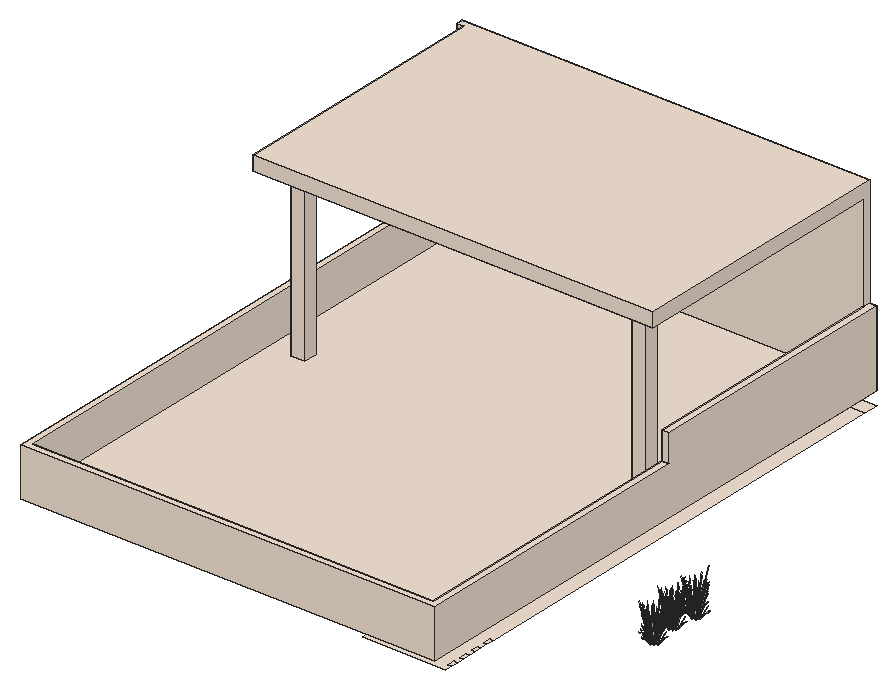
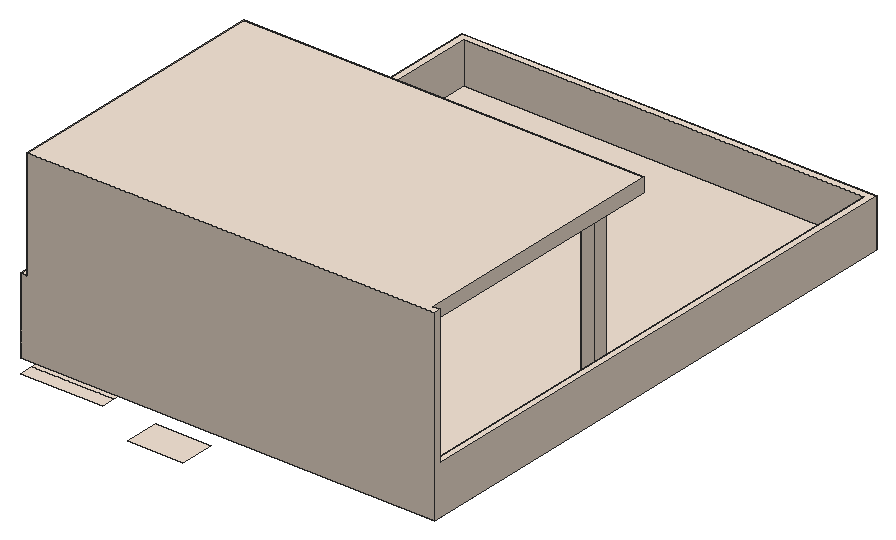
# SketchUp Ruby script. Lengths in inches.
U = 1.inch
M = Sketchup.active_model
def pt(a) = Geom::Point3d.new(a.map { |v| v * U })
def face(e, loops, mat)
  f = e.add_face(loops[0].map { |a| pt(a) })
  loops[1..].each { |l| e.add_face(l.map { |a| pt(a) }).erase! }
  f.material = f.back_material = mat if mat
  f
end
# faces: each face lists its corners as indices into pts; further lists are holes
def faces(e, pts, list, mat = nil) = list.each { |f| face(e, (f[0].is_a?(Array) ? f : [f]).map { |l| l.map { |i| pts[i] } }, mat) }
# xy, xz, yz: faces in a plane at the given z, y or x. An outline is a flat list of corners, or four numbers for a rectangle; further outlines are holes
def ring(l) = l.size == 4 ? [[l[0], l[1]], [l[2], l[1]], [l[2], l[3]], [l[0], l[3]]] : l.each_slice(2).to_a
def flat(e, list, mat, &to3) = list.each { |f| face(e, (f[0].is_a?(Array) ? f : [f]).map { |l| ring(l).map { |u, v| to3.(u, v) } }, mat) }
def xy(e, z, list, mat = nil) = flat(e, list, mat) { |x, y| [x, y, z] }
def xz(e, y, list, mat = nil) = flat(e, list, mat) { |x, z| [x, y, z] }
def yz(e, x, list, mat = nil) = flat(e, list, mat) { |y, z| [x, y, z] }
def lines(e, pts, list) = list.each { |a, b| e.add_line(pt(pts[a]), pt(pts[b])) }
# prism: a flat outline (further loops are holes) pulled along v
def prism(e, loops, v, mat = nil)
  f = face(e, loops, mat); d = Geom::Vector3d.new(v.map { |x| x * U })
  f.pushpull(f.normal.samedirection?(d) ? d.length : -d.length)
end
def box(e, o, s, mat = nil) = prism(e, [[o, [o[0] + s[0], o[1], o[2]], [o[0] + s[0], o[1] + s[1], o[2]], [o[0], o[1] + s[1], o[2]]]], [0, 0, s[2]], mat)
def at(x, y, z, deg = 0) = Geom::Transformation.translation(pt([x, y, z])) * Geom::Transformation.rotation(ORIGIN, Z_AXIS, deg.degrees)
def axes(o, x, y, z) = Geom::Transformation.new([*x, 0, *y, 0, *z, 0, *pt(o).to_a, 1])
def part(name) = M.definitions.add(name)
# library, detail: a bought-in or finely detailed component or shape, given as its bounding box
def library(name, o, s) = part(name).tap { |d| box(d.entities, o, s) }
def detail(e, o, s) = box(e.add_group.entities, o, s)
def put(e, d, t, mat = nil) = e.add_instance(d, t).tap { |i| i.material = mat if mat }
def group(e, t, mat = nil) = e.add_group.tap { |g| g.transformation = t; g.material = mat if mat }.entities
root = M.entities
M.materials.add("C01_Vanilla_Cream").color = [244, 228, 212]
M.materials.add("LightPink_Translucent").color = [144, 107, 117]
M.materials["LightPink_Translucent"].alpha = 0.75
c1 = part("blade")
p = [[2.15,0.21,22],[0,0.17,0],[0.09,0.45,0],[2.18,0.31,22],[2.29,0.31,22],[0.38,0.45,0],
  [2.48,0.24,33],[2.49,0.24,33],[2.48,0.22,33]]
faces(c1.entities,p,[[0,1,2,3],[4,5,2,3],[6,3,4,7],[8,0,3,6]])
c2 = part("seeds")
p = [[0.3,-0.1,1.38],[-0.01,-0.03,1.59],[-0.01,-0.03,0.03],[0.14,-0.07,-0.07],[0.29,-0.03,3],[0.15,0.01,3.11]]
faces(c2.entities,p,[[0,1,2,3],[1,0,4,5]],"LightPink_Translucent")
c3 = part("blade with seeds")
put(c3.entities,c1,at(0,0,0))
put(c3.entities,c2,axes([2.4,0.25,30.99],[1.5799,-0.05474,1.17369],[-0.12525,1.92788,0.29478],[-0.07173,-0.02425,1.56792]))
xy(root,543,[[226.53,171,288,201],[240,327,290,358.5],[240,361.5,290,393],[240,423,288,453]],"C01_Vanilla_Cream")
xy(root,546,[[288,324,290,396]],"C01_Vanilla_Cream")
xy(root,582,[[288,12,288,216,326.85,216,326.85,314.71,288,314.71,288,468,360,468,360,63.65,357,63.65,357,57.2,360,57.2,360,50.74,357,50.74,357,44.28,360,44.28,360,37.83,357,37.83,357,31.37,360,31.37,360,24.91,357,24.91,357,18.46,360,18.46,360,12],[357,18.46,360,24.91],[357,31.37,360,37.83],[357,44.28,360,50.74],[357,57.2,360,63.65],
  [288,468,360,480]],"C01_Vanilla_Cream")
xy(root,594,[[[0,0,360,480],[9,9,351,471]]],"C01_Vanilla_Cream")
p = [[360,254.66,636],[354,254.66,636]]
lines(root,p,[[0,1]])
put(root,c3,axes([356.1,285.38,501.78],[-0.02981,0.50103,-0.0912],[-0.56442,-0.01369,-0.50621],[-0.21738,-0.0348,0.76918]))
put(root,c3,axes([358.58,288.78,501.78],[0.33176,-0.4217,-0.0912],[0.48044,0.24295,-0.50621],[0.16701,0.11914,0.76918]))
put(root,c3,axes([355.49,287.37,501.78],[0.515,0.27165,-0.0912],[-0.2967,0.3934,-0.50621],[-0.1455,0.13675,0.76918]))
put(root,c3,axes([358.5,284.82,501.78],[-0.54481,0.22937,-0.0912],[-0.26773,-0.4071,-0.50621],[-0.07188,-0.17155,0.76918]))
put(root,c3,axes([360.3,286.25,501.78],[-0.515,-0.27165,-0.0912],[0.2967,-0.3934,-0.50621],[0.1455,-0.13675,0.76918]))
put(root,c3,axes([358.96,240.81,501.36],[-0.48108,-0.25598,1.03712],[0.50798,-0.39855,0.44749],[0.15521,0.24018,1.00248]))
put(root,c3,axes([355.92,264.77,501.36],[-0.48108,-0.25598,1.03712],[0.50798,-0.39855,0.44749],[0.15521,0.24018,1.00248]))
put(root,c3,axes([358.96,286.29,501.36],[-0.48108,-0.25598,1.03712],[0.50798,-0.39855,0.44749],[0.15521,0.24018,1.00248]))
put(root,c3,axes([354.88,241.27,501.54],[-0.09091,0.06396,1.31208],[0.00773,0.46734,-0.2075],[-0.20839,0.06078,0.10523]))
put(root,c3,axes([361.84,241.125,501.54],[0.07726,-0.07504,1.31208],[-0.09888,-0.46032,-0.2075],[0.19384,-0.08728,0.10523]))
put(root,c3,axes([360.18,242.45,501.54],[0.11943,-0.00833,1.31208],[0.32759,-0.38275,-0.2075],[0.21244,0.05052,0.10523]))
put(root,c3,axes([360.19,239.12,501.54],[-0.00537,-0.09805,1.31208],[-0.45391,-0.28338,-0.2075],[0.07018,-0.17178,0.10523]))
put(root,c3,axes([354.9,243.02,501.54],[-0.01384,0.09749,1.31208],[0.39274,0.33916,-0.2075],[-0.10282,0.16039,0.10523]))
put(root,c3,axes([357.16,244.22,501.54],[0.07057,0.07933,1.31208],[0.56952,0.03117,-0.2075],[0.05727,0.17496,0.10523]))
put(root,c3,axes([357.64,238.27,501.54],[-0.08515,-0.06907,1.31208],[-0.56828,0.04379,-0.2075],[-0.0907,-0.16522,0.10523]))
put(root,c3,axes([355.77,239.03,501.54],[-0.11979,-0.00348,1.31208],[-0.38137,0.34775,-0.2075],[-0.20349,-0.07106,0.10523]))
put(root,c3,axes([351.85,265.24,501.54],[-0.09091,0.06396,1.31208],[0.00773,0.46734,-0.2075],[-0.20839,0.06078,0.10523]))
put(root,c3,axes([358.8,265.09,501.54],[0.07726,-0.07504,1.31208],[-0.09888,-0.46032,-0.2075],[0.19384,-0.08728,0.10523]))
put(root,c3,axes([357.14,266.42,501.54],[0.11943,-0.00833,1.31208],[0.32759,-0.38275,-0.2075],[0.21244,0.05052,0.10523]))
put(root,c3,axes([357.15,263.08,501.54],[-0.00537,-0.09805,1.31208],[-0.45391,-0.28338,-0.2075],[0.07018,-0.17178,0.10523]))
put(root,c3,axes([351.86,266.98,501.54],[-0.01384,0.09749,1.31208],[0.39274,0.33916,-0.2075],[-0.10282,0.16039,0.10523]))
put(root,c3,axes([354.12,268.1875,501.54],[0.07057,0.07933,1.31208],[0.56952,0.03117,-0.2075],[0.05727,0.17496,0.10523]))
put(root,c3,axes([354.6,262.24,501.54],[-0.08515,-0.06907,1.31208],[-0.56828,0.04379,-0.2075],[-0.0907,-0.16522,0.10523]))
put(root,c3,axes([352.74,263,501.54],[-0.11979,-0.00348,1.31208],[-0.38137,0.34775,-0.2075],[-0.20349,-0.07106,0.10523]))
put(root,c3,axes([354.88,286.76,501.54],[-0.09091,0.06396,1.31208],[0.00773,0.46734,-0.2075],[-0.20839,0.06078,0.10523]))
put(root,c3,axes([361.84,286.61,501.54],[0.07726,-0.07504,1.31208],[-0.09888,-0.46032,-0.2075],[0.19384,-0.08728,0.10523]))
put(root,c3,axes([360.18,287.93,501.54],[0.11943,-0.00833,1.31208],[0.32759,-0.38275,-0.2075],[0.21244,0.05052,0.10523]))
put(root,c3,axes([360.19,284.6,501.54],[-0.00537,-0.09805,1.31208],[-0.45391,-0.28338,-0.2075],[0.07018,-0.17178,0.10523]))
put(root,c3,axes([354.9,288.5,501.54],[-0.01384,0.09749,1.31208],[0.39274,0.33916,-0.2075],[-0.10282,0.16039,0.10523]))
put(root,c3,axes([357.16,289.71,501.54],[0.07057,0.07933,1.31208],[0.56952,0.03117,-0.2075],[0.05727,0.17496,0.10523]))
put(root,c3,axes([357.64,283.76,501.54],[-0.08515,-0.06907,1.31208],[-0.56828,0.04379,-0.2075],[-0.0907,-0.16522,0.10523]))
put(root,c3,axes([355.77,284.52,501.54],[-0.11979,-0.00348,1.31208],[-0.38137,0.34775,-0.2075],[-0.20349,-0.07106,0.10523]))
put(root,c3,axes([355.3125,239.33,501.53],[0.04127,0.04917,1.33037],[-0.19898,0.44196,-0.12571],[-0.20151,0.0032,0.23543]))
put(root,c3,axes([357.05,238.05,501.53],[-0.01039,0.05905,1.33037],[-0.51226,0.21431,-0.12571],[-0.15074,-0.10955,0.23543]))
put(root,c3,axes([358.15,243.64,501.53],[0.00165,-0.05965,1.33037],[0.47711,-0.26315,-0.12571],[0.16572,0.09393,0.23543]))
put(root,c3,axes([353.87,241.74,501.53],[0.07105,0.01321,1.33037],[0.2198,0.43529,-0.12571],[-0.14545,0.11425,0.23543]))
put(root,c3,axes([361.57,240.64,501.53],[-0.07272,-0.00374,1.33037],[-0.30197,-0.40092,-0.12571],[0.12127,-0.13182,0.23543]))
put(root,c3,axes([361.44,243.15,501.53],[-0.05034,-0.04313,1.33037],[0.11012,-0.46232,-0.12571],[0.1983,-0.02954,0.23543]))
put(root,c3,axes([354.85,244.02,501.53],[0.06316,-0.02974,1.33037],[0.52204,0.19785,-0.12571],[-0.01227,0.16473,0.23543]))
put(root,c3,axes([360.07,238.77,501.53],[-0.05654,0.03763,1.33037],[-0.55396,-0.12696,-0.12571],[-0.02005,-0.16422,0.23543]))
put(root,c3,axes([352.28,263.29,501.53],[0.04127,0.04917,1.33037],[-0.19898,0.44196,-0.12571],[-0.20151,0.0032,0.23543]))
put(root,c3,axes([354.02,262.01,501.53],[-0.01039,0.05905,1.33037],[-0.51226,0.21431,-0.12571],[-0.15074,-0.10955,0.23543]))
put(root,c3,axes([355.11,267.61,501.53],[0.00165,-0.05965,1.33037],[0.47711,-0.26315,-0.12571],[0.16572,0.09393,0.23543]))
put(root,c3,axes([350.84,265.71,501.53],[0.07105,0.01321,1.33037],[0.2198,0.43529,-0.12571],[-0.14545,0.11425,0.23543]))
put(root,c3,axes([358.53,264.61,501.53],[-0.07272,-0.00374,1.33037],[-0.30197,-0.40092,-0.12571],[0.12127,-0.13182,0.23543]))
put(root,c3,axes([358.4,267.11,501.53],[-0.05034,-0.04313,1.33037],[0.11012,-0.46232,-0.12571],[0.1983,-0.02954,0.23543]))
put(root,c3,axes([351.82,267.98,501.53],[0.06316,-0.02974,1.33037],[0.52204,0.19785,-0.12571],[-0.01227,0.16473,0.23543]))
put(root,c3,axes([357.03,262.73,501.53],[-0.05654,0.03763,1.33037],[-0.55396,-0.12696,-0.12571],[-0.02005,-0.16422,0.23543]))
put(root,c3,axes([355.3125,284.8125,501.53],[0.04127,0.04917,1.33037],[-0.19898,0.44196,-0.12571],[-0.20151,0.0032,0.23543]))
put(root,c3,axes([357.05,283.53,501.53],[-0.01039,0.05905,1.33037],[-0.51226,0.21431,-0.12571],[-0.15074,-0.10955,0.23543]))
put(root,c3,axes([358.15,289.13,501.53],[0.00165,-0.05965,1.33037],[0.47711,-0.26315,-0.12571],[0.16572,0.09393,0.23543]))
put(root,c3,axes([353.87,287.23,501.53],[0.07105,0.01321,1.33037],[0.2198,0.43529,-0.12571],[-0.14545,0.11425,0.23543]))
put(root,c3,axes([361.57,286.13,501.53],[-0.07272,-0.00374,1.33037],[-0.30197,-0.40092,-0.12571],[0.12127,-0.13182,0.23543]))
put(root,c3,axes([361.44,288.63,501.53],[-0.05034,-0.04313,1.33037],[0.11012,-0.46232,-0.12571],[0.1983,-0.02954,0.23543]))
put(root,c3,axes([354.85,289.5,501.53],[0.06316,-0.02974,1.33037],[0.52204,0.19785,-0.12571],[-0.01227,0.16473,0.23543]))
put(root,c3,axes([360.07,284.25,501.53],[-0.05654,0.03763,1.33037],[-0.55396,-0.12696,-0.12571],[-0.02005,-0.16422,0.23543]))
put(root,c3,axes([356.15,242.8,502.05],[0.61188,0.02441,-0.10123],[-0.01672,0.46217,-0.56189],[-0.0425,0.178,0.85379]))
put(root,c3,axes([353.12,266.76,502.05],[0.61188,0.02441,-0.10123],[-0.01672,0.46217,-0.56189],[-0.0425,0.178,0.85379]))
put(root,c3,axes([356.15,288.28,502.05],[0.61188,0.02441,-0.10123],[-0.01672,0.46217,-0.56189],[-0.0425,0.178,0.85379]))
put(root,c3,axes([357.2,239.17,502.07],[-0.37157,0.4723,-0.10215],[-0.5381,-0.2721,-0.56695],[-0.18705,-0.13344,0.86148]))
put(root,c3,axes([354.16,263.13,502.07],[-0.37157,0.4723,-0.10215],[-0.5381,-0.2721,-0.56695],[-0.18705,-0.13344,0.86148]))
put(root,c3,axes([357.2,284.65,502.07],[-0.37157,0.4723,-0.10215],[-0.5381,-0.2721,-0.56695],[-0.18705,-0.13344,0.86148]))
put(root,c3,axes([357.08,239.2,501.55],[0.25304,-0.31296,0.04823],[0.36033,0.18221,0.37966],[-0.11649,-0.10034,0.57892]))
put(root,c3,axes([357.3,243.5,501.55],[-0.41024,0.16744,0.04823],[-0.2008,-0.30532,0.37966],[0.03962,0.13459,0.57892]))
put(root,c3,axes([360.49,240.66,501.55],[0.3822,0.20719,0.04823],[-0.22252,0.29505,0.37966],[0.12254,-0.09539,0.57892]))
put(root,c3,axes([360.55,241.8125,501.55],[0.20448,0.33592,0.04823],[-0.37288,0.16442,0.37966],[0.16437,-0.03244,0.57892]))
put(root,c3,axes([355.9,239.82,501.55],[0.02803,-0.37463,0.04823],[0.42332,0.01027,0.37966],[-0.16216,-0.0392,0.57892]))
put(root,c3,axes([359.74,239.6875,501.55],[0.45752,0.02296,0.04823],[-0.01254,0.34663,0.37966],[0.04787,-0.13278,0.57892]))
put(root,c3,axes([359.89,242.83,501.55],[-0.02803,0.37463,0.04823],[-0.42332,-0.01027,0.37966],[0.16216,0.0392,0.57892]))
put(root,c3,axes([355.3,241.99,501.55],[-0.3822,-0.20719,0.04823],[0.22252,-0.29505,0.37966],[-0.12254,0.09539,0.57892]))
put(root,c3,axes([358.49,239.15,501.55],[0.41024,-0.16744,0.04823],[0.2008,0.30532,0.37966],[-0.03962,-0.13459,0.57892]))
put(root,c3,axes([355.24,240.84,501.55],[-0.20448,-0.33592,0.04823],[0.37288,-0.16442,0.37966],[-0.16437,0.03244,0.57892]))
put(root,c3,axes([358.7,243.45,501.55],[-0.25304,0.31296,0.04823],[-0.36033,-0.18221,0.37966],[0.11649,0.10034,0.57892]))
put(root,c3,axes([356.05,242.96,501.55],[-0.45752,-0.02296,0.04823],[0.01254,-0.34663,0.37966],[-0.04787,0.13278,0.57892]))
put(root,c3,axes([354.05,263.17,501.55],[0.25304,-0.31296,0.04823],[0.36033,0.18221,0.37966],[-0.11649,-0.10034,0.57892]))
put(root,c3,axes([354.26,267.46,501.55],[-0.41024,0.16744,0.04823],[-0.2008,-0.30532,0.37966],[0.03962,0.13459,0.57892]))
put(root,c3,axes([357.45,264.63,501.55],[0.3822,0.20719,0.04823],[-0.22252,0.29505,0.37966],[0.12254,-0.09539,0.57892]))
put(root,c3,axes([357.51,265.78,501.55],[0.20448,0.33592,0.04823],[-0.37288,0.16442,0.37966],[0.16437,-0.03244,0.57892]))
put(root,c3,axes([352.86,263.78,501.55],[0.02803,-0.37463,0.04823],[0.42332,0.01027,0.37966],[-0.16216,-0.0392,0.57892]))
put(root,c3,axes([356.7,263.66,501.55],[0.45752,0.02296,0.04823],[-0.01254,0.34663,0.37966],[0.04787,-0.13278,0.57892]))
put(root,c3,axes([356.85,266.8,501.55],[-0.02803,0.37463,0.04823],[-0.42332,-0.01027,0.37966],[0.16216,0.0392,0.57892]))
put(root,c3,axes([352.26,265.95,501.55],[-0.3822,-0.20719,0.04823],[0.22252,-0.29505,0.37966],[-0.12254,0.09539,0.57892]))
put(root,c3,axes([355.45,263.12,501.55],[0.41024,-0.16744,0.04823],[0.2008,0.30532,0.37966],[-0.03962,-0.13459,0.57892]))
put(root,c3,axes([352.21,264.8,501.55],[-0.20448,-0.33592,0.04823],[0.37288,-0.16442,0.37966],[-0.16437,0.03244,0.57892]))
put(root,c3,axes([355.67,267.42,501.55],[-0.25304,0.31296,0.04823],[-0.36033,-0.18221,0.37966],[0.11649,0.10034,0.57892]))
put(root,c3,axes([353.01,266.93,501.55],[-0.45752,-0.02296,0.04823],[0.01254,-0.34663,0.37966],[-0.04787,0.13278,0.57892]))
put(root,c3,axes([357.08,284.69,501.55],[0.25304,-0.31296,0.04823],[0.36033,0.18221,0.37966],[-0.11649,-0.10034,0.57892]))
put(root,c3,axes([357.3,288.98,501.55],[-0.41024,0.16744,0.04823],[-0.2008,-0.30532,0.37966],[0.03962,0.13459,0.57892]))
put(root,c3,axes([360.49,286.15,501.55],[0.3822,0.20719,0.04823],[-0.22252,0.29505,0.37966],[0.12254,-0.09539,0.57892]))
put(root,c3,axes([360.55,287.3,501.55],[0.20448,0.33592,0.04823],[-0.37288,0.16442,0.37966],[0.16437,-0.03244,0.57892]))
put(root,c3,axes([355.9,285.3,501.55],[0.02803,-0.37463,0.04823],[0.42332,0.01027,0.37966],[-0.16216,-0.0392,0.57892]))
put(root,c3,axes([359.74,285.17,501.55],[0.45752,0.02296,0.04823],[-0.01254,0.34663,0.37966],[0.04787,-0.13278,0.57892]))
put(root,c3,axes([359.89,288.32,501.55],[-0.02803,0.37463,0.04823],[-0.42332,-0.01027,0.37966],[0.16216,0.0392,0.57892]))
put(root,c3,axes([355.3,287.47,501.55],[-0.3822,-0.20719,0.04823],[0.22252,-0.29505,0.37966],[-0.12254,0.09539,0.57892]))
put(root,c3,axes([358.49,284.64,501.55],[0.41024,-0.16744,0.04823],[0.2008,0.30532,0.37966],[-0.03962,-0.13459,0.57892]))
put(root,c3,axes([355.24,286.32,501.55],[-0.20448,-0.33592,0.04823],[0.37288,-0.16442,0.37966],[-0.16437,0.03244,0.57892]))
put(root,c3,axes([358.7,288.93,501.55],[-0.25304,0.31296,0.04823],[-0.36033,-0.18221,0.37966],[0.11649,0.10034,0.57892]))
put(root,c3,axes([356.05,288.45,501.55],[-0.45752,-0.02296,0.04823],[0.01254,-0.34663,0.37966],[-0.04787,0.13278,0.57892]))
put(root,c3,axes([358.34,239.1875,501.55],[0.54859,0.1288,0.36002],[-0.18759,0.42344,0.29685],[-0.03297,-0.16652,0.74497]))
put(root,c3,axes([359.93,242.71,501.55],[-0.41051,0.32462,0.36002],[-0.35404,-0.34474,0.29685],[0.1926,0.05988,0.74497]))
put(root,c3,axes([360.51,241.69,501.55],[-0.15729,0.44921,0.36002],[-0.51712,-0.15361,0.29685],[0.20336,-0.027,0.74497]))
put(root,c3,axes([355.41,242.07,501.55],[-0.13808,-0.45342,0.36002],[0.54163,-0.07869,0.29685],[-0.15963,0.10664,0.74497]))
put(root,c3,axes([356.2,242.99,501.55],[-0.39645,-0.33614,0.36002],[0.42102,-0.2899,0.29685],[-0.07313,0.15771,0.74497]))
put(root,c3,axes([359.59,239.66,501.55],[0.39645,0.33614,0.36002],[-0.42102,0.2899,0.29685],[0.07313,-0.15771,0.74497]))
put(root,c3,axes([355.28,240.96,501.55],[0.15729,-0.44921,0.36002],[0.51712,0.15361,0.29685],[-0.20336,0.027,0.74497]))
put(root,c3,axes([360.38,240.57,501.55],[0.13808,0.45342,0.36002],[-0.54163,0.07869,0.29685],[0.15963,-0.10664,0.74497]))
put(root,c3,axes([358.81,243.36,501.55],[-0.55374,0.11306,0.36002],[-0.0961,-0.44351,0.29685],[0.13023,0.13071,0.74497]))
put(root,c3,axes([355.31,263.15,501.55],[0.54859,0.1288,0.36002],[-0.18759,0.42344,0.29685],[-0.03297,-0.16652,0.74497]))
put(root,c3,axes([356.89,266.68,501.55],[-0.41051,0.32462,0.36002],[-0.35404,-0.34474,0.29685],[0.1926,0.05988,0.74497]))
put(root,c3,axes([357.47,265.66,501.55],[-0.15729,0.44921,0.36002],[-0.51712,-0.15361,0.29685],[0.20336,-0.027,0.74497]))
put(root,c3,axes([352.37,266.04,501.55],[-0.13808,-0.45342,0.36002],[0.54163,-0.07869,0.29685],[-0.15963,0.10664,0.74497]))
put(root,c3,axes([353.16,266.96,501.55],[-0.39645,-0.33614,0.36002],[0.42102,-0.2899,0.29685],[-0.07313,0.15771,0.74497]))
put(root,c3,axes([356.55,263.625,501.55],[0.39645,0.33614,0.36002],[-0.42102,0.2899,0.29685],[0.07313,-0.15771,0.74497]))
put(root,c3,axes([352.24,264.92,501.55],[0.15729,-0.44921,0.36002],[0.51712,0.15361,0.29685],[-0.20336,0.027,0.74497]))
put(root,c3,axes([357.34,264.54,501.55],[0.13808,0.45342,0.36002],[-0.54163,0.07869,0.29685],[0.15963,-0.10664,0.74497]))
put(root,c3,axes([355.77,267.33,501.55],[-0.55374,0.11306,0.36002],[-0.0961,-0.44351,0.29685],[0.13023,0.13071,0.74497]))
put(root,c3,axes([358.34,284.67,501.55],[0.54859,0.1288,0.36002],[-0.18759,0.42344,0.29685],[-0.03297,-0.16652,0.74497]))
put(root,c3,axes([359.93,288.2,501.55],[-0.41051,0.32462,0.36002],[-0.35404,-0.34474,0.29685],[0.1926,0.05988,0.74497]))
put(root,c3,axes([360.51,287.18,501.55],[-0.15729,0.44921,0.36002],[-0.51712,-0.15361,0.29685],[0.20336,-0.027,0.74497]))
put(root,c3,axes([355.41,287.56,501.55],[-0.13808,-0.45342,0.36002],[0.54163,-0.07869,0.29685],[-0.15963,0.10664,0.74497]))
put(root,c3,axes([356.2,288.48,501.55],[-0.39645,-0.33614,0.36002],[0.42102,-0.2899,0.29685],[-0.07313,0.15771,0.74497]))
put(root,c3,axes([359.59,285.14,501.55],[0.39645,0.33614,0.36002],[-0.42102,0.2899,0.29685],[0.07313,-0.15771,0.74497]))
put(root,c3,axes([355.28,286.44,501.55],[0.15729,-0.44921,0.36002],[0.51712,0.15361,0.29685],[-0.20336,0.027,0.74497]))
put(root,c3,axes([360.38,286.06,501.55],[0.13808,0.45342,0.36002],[-0.54163,0.07869,0.29685],[0.15963,-0.10664,0.74497]))
put(root,c3,axes([358.81,288.85,501.55],[-0.55374,0.11306,0.36002],[-0.0961,-0.44351,0.29685],[0.13023,0.13071,0.74497]))
put(root,c3,axes([357.45,243.15,501.79],[0.16784,-0.37886,0.2656],[0.48968,0.1105,-0.3429],[0.0449,0.15254,0.65611]))
put(root,c3,axes([358.34,239.5,501.79],[-0.16784,0.37886,0.2656],[-0.48968,-0.1105,-0.3429],[-0.0449,-0.15254,0.65611]))
put(root,c3,axes([359.6,242.55,501.79],[-0.31678,-0.30846,0.2656],[0.36171,-0.29199,-0.3429],[0.18378,0.04443,0.65611]))
put(root,c3,axes([360.125,241.6875,501.79],[-0.46269,-0.13744,0.2656],[0.13495,-0.40096,-0.3429],[0.18628,-0.03677,0.65611]))
put(root,c3,axes([356.18,240.1,501.79],[0.31678,0.30846,0.2656],[-0.36171,0.29199,-0.3429],[-0.18378,-0.04443,0.65611]))
put(root,c3,axes([356.39,242.73,501.79],[0.3767,-0.25939,0.2656],[0.3566,0.29618,-0.3429],[-0.05426,0.15048,0.65611]))
put(root,c3,axes([355.74,241.92,501.79],[0.48462,-0.07041,0.2656],[0.12797,0.4025,-0.3429],[-0.13888,0.10811,0.65611]))
put(root,c3,axes([358.625,243.09,501.79],[-0.08599,-0.39682,0.2656],[0.49155,-0.10478,-0.3429],[0.13203,0.11372,0.65611]))
put(root,c3,axes([360.05,240.73,501.79],[-0.48462,0.07041,0.2656],[-0.12797,-0.4025,-0.3429],[0.13888,-0.10811,0.65611]))
put(root,c3,axes([355.66,240.96,501.79],[0.46269,0.13744,0.2656],[-0.13495,0.40096,-0.3429],[-0.18628,0.03677,0.65611]))
put(root,c3,axes([359.39,239.92,501.79],[-0.3767,0.25939,0.2656],[-0.3566,-0.29618,-0.3429],[0.05426,-0.15048,0.65611]))
put(root,c3,axes([357.16,239.56,501.79],[0.08599,0.39682,0.2656],[-0.49155,0.10478,-0.3429],[-0.13203,-0.11372,0.65611]))
put(root,c3,axes([354.41,267.12,501.79],[0.16784,-0.37886,0.2656],[0.48968,0.1105,-0.3429],[0.0449,0.15254,0.65611]))
put(root,c3,axes([355.3,263.46,501.79],[-0.16784,0.37886,0.2656],[-0.48968,-0.1105,-0.3429],[-0.0449,-0.15254,0.65611]))
put(root,c3,axes([356.57,266.52,501.79],[-0.31678,-0.30846,0.2656],[0.36171,-0.29199,-0.3429],[0.18378,0.04443,0.65611]))
put(root,c3,axes([357.09,265.65,501.79],[-0.46269,-0.13744,0.2656],[0.13495,-0.40096,-0.3429],[0.18628,-0.03677,0.65611]))
put(root,c3,axes([353.15,264.0625,501.79],[0.31678,0.30846,0.2656],[-0.36171,0.29199,-0.3429],[-0.18378,-0.04443,0.65611]))
put(root,c3,axes([353.36,266.69,501.79],[0.3767,-0.25939,0.2656],[0.3566,0.29618,-0.3429],[-0.05426,0.15048,0.65611]))
put(root,c3,axes([352.7,265.89,501.79],[0.48462,-0.07041,0.2656],[0.12797,0.4025,-0.3429],[-0.13888,0.10811,0.65611]))
put(root,c3,axes([355.59,267.06,501.79],[-0.08599,-0.39682,0.2656],[0.49155,-0.10478,-0.3429],[0.13203,0.11372,0.65611]))
put(root,c3,axes([357.01,264.69,501.79],[-0.48462,0.07041,0.2656],[-0.12797,-0.4025,-0.3429],[0.13888,-0.10811,0.65611]))
put(root,c3,axes([352.625,264.93,501.79],[0.46269,0.13744,0.2656],[-0.13495,0.40096,-0.3429],[-0.18628,0.03677,0.65611]))
put(root,c3,axes([356.36,263.89,501.79],[-0.3767,0.25939,0.2656],[-0.3566,-0.29618,-0.3429],[0.05426,-0.15048,0.65611]))
put(root,c3,axes([354.125,263.53,501.79],[0.08599,0.39682,0.2656],[-0.49155,0.10478,-0.3429],[-0.13203,-0.11372,0.65611]))
put(root,c3,axes([357.45,288.64,501.79],[0.16784,-0.37886,0.2656],[0.48968,0.1105,-0.3429],[0.0449,0.15254,0.65611]))
put(root,c3,axes([358.34,284.98,501.79],[-0.16784,0.37886,0.2656],[-0.48968,-0.1105,-0.3429],[-0.0449,-0.15254,0.65611]))
put(root,c3,axes([359.6,288.04,501.79],[-0.31678,-0.30846,0.2656],[0.36171,-0.29199,-0.3429],[0.18378,0.04443,0.65611]))
put(root,c3,axes([360.125,287.17,501.79],[-0.46269,-0.13744,0.2656],[0.13495,-0.40096,-0.3429],[0.18628,-0.03677,0.65611]))
put(root,c3,axes([356.18,285.58,501.79],[0.31678,0.30846,0.2656],[-0.36171,0.29199,-0.3429],[-0.18378,-0.04443,0.65611]))
put(root,c3,axes([356.39,288.21,501.79],[0.3767,-0.25939,0.2656],[0.3566,0.29618,-0.3429],[-0.05426,0.15048,0.65611]))
put(root,c3,axes([355.74,287.41,501.79],[0.48462,-0.07041,0.2656],[0.12797,0.4025,-0.3429],[-0.13888,0.10811,0.65611]))
put(root,c3,axes([358.625,288.57,501.79],[-0.08599,-0.39682,0.2656],[0.49155,-0.10478,-0.3429],[0.13203,0.11372,0.65611]))
put(root,c3,axes([360.05,286.21,501.79],[-0.48462,0.07041,0.2656],[-0.12797,-0.4025,-0.3429],[0.13888,-0.10811,0.65611]))
put(root,c3,axes([355.66,286.45,501.79],[0.46269,0.13744,0.2656],[-0.13495,0.40096,-0.3429],[-0.18628,0.03677,0.65611]))
put(root,c3,axes([359.39,285.41,501.79],[-0.3767,0.25939,0.2656],[-0.3566,-0.29618,-0.3429],[0.05426,-0.15048,0.65611]))
put(root,c3,axes([357.16,285.05,501.79],[0.08599,0.39682,0.2656],[-0.49155,0.10478,-0.3429],[-0.13203,-0.11372,0.65611]))
put(root,c3,axes([357.44,243.46,501.8],[-0.54859,-0.1288,0.39962],[0.18759,-0.42344,0.32951],[0.03297,0.16652,0.82692]))
put(root,c3,axes([354.41,267.43,501.8],[-0.54859,-0.1288,0.39962],[0.18759,-0.42344,0.32951],[0.03297,0.16652,0.82692]))
put(root,c3,axes([357.44,288.95,501.8],[-0.54859,-0.1288,0.39962],[0.18759,-0.42344,0.32951],[0.03297,0.16652,0.82692]))
put(root,c3,axes([355.6875,239.82,501.82],[0.45978,-0.36358,0.40322],[0.39653,0.38611,0.33247],[-0.21571,-0.06707,0.83437]))
put(root,c3,axes([356.94,239.09,501.82],[0.62019,-0.12663,0.40322],[0.10763,0.49673,0.33247],[-0.14586,-0.1464,0.83437]))
put(root,c3,axes([352.65,263.79,501.82],[0.45978,-0.36358,0.40322],[0.39653,0.38611,0.33247],[-0.21571,-0.06707,0.83437]))
put(root,c3,axes([353.9,263.06,501.82],[0.62019,-0.12663,0.40322],[0.10763,0.49673,0.33247],[-0.14586,-0.1464,0.83437]))
put(root,c3,axes([355.6875,285.3,501.82],[0.45978,-0.36358,0.40322],[0.39653,0.38611,0.33247],[-0.21571,-0.06707,0.83437]))
put(root,c3,axes([356.94,284.58,501.82],[0.62019,-0.12663,0.40322],[0.10763,0.49673,0.33247],[-0.14586,-0.1464,0.83437]))
put(root,c3,axes([358.11,244.5,502.23],[0.38473,-0.28263,-0.04866],[0.35252,0.30954,-0.22062],[0.02482,0.08771,0.72768]))
put(root,c3,axes([354.64,243.07,502.23],[0.49129,0.13151,-0.04866],[-0.15113,0.40475,-0.22062],[-0.08035,0.06145,0.72768]))
put(root,c3,axes([355.07,268.47,502.23],[0.38473,-0.28263,-0.04866],[0.35252,0.30954,-0.22062],[0.02482,0.08771,0.72768]))
put(root,c3,axes([351.6,267.03,502.23],[0.49129,0.13151,-0.04866],[-0.15113,0.40475,-0.22062],[-0.08035,0.06145,0.72768]))
put(root,c3,axes([358.11,289.99,502.23],[0.38473,-0.28263,-0.04866],[0.35252,0.30954,-0.22062],[0.02482,0.08771,0.72768]))
put(root,c3,axes([354.64,288.55,502.23],[0.49129,0.13151,-0.04866],[-0.15113,0.40475,-0.22062],[-0.08035,0.06145,0.72768]))
g1 = group(root,at(0,0,594),"C01_Vanilla_Cream")
xy(g1,0,[[0,0,360,480]])
xy(g1,6,[[[6,6,354,474],[323.13,260.72,335.13,272.72],[26.31,260.72,38.31,272.72]]])
xy(g1,42,[[0,0,360,0,360,254.66,354,254.66,354,6,6,6,6,474,0,474]])
xy(g1,66,[[354,254.66,360,480]])
xy(g1,150,[[[6,244.9,354,474],[323.13,260.72,335.13,272.72],[26.31,260.72,38.31,272.72]]])
xy(g1,156,[[26.31,260.72,38.31,272.72],[323.13,260.72,335.13,272.72]])
xy(g1,162,[[6,244.9,354,244.9,354,480,0,480,0,474,6,474]])
xz(g1,0,[[0,0,360,42]])
xz(g1,6,[[6,6,354,42]])
xz(g1,244.9,[[6,150,354,162]])
xz(g1,254.66,[[354,42,360,66]])
xz(g1,260.72,[[26.31,6,38.31,150],[323.13,6,335.13,150],[26.31,150,38.31,156],[323.13,150,335.13,156]])
xz(g1,272.72,[[26.31,6,38.31,150],[323.13,6,335.13,150],[26.31,150,38.31,156],[323.13,150,335.13,156]])
xz(g1,474,[[6,6,354,150],[0,42,6,162]])
xz(g1,480,[[0,0,0,162,354,162,354,66,360,66,360,0]])
yz(g1,0,[[0,0,0,42,474,42,474,162,480,162,480,0]])
yz(g1,6,[[6,6,474,42],[244.9,150,474,162]])
yz(g1,26.31,[[260.72,6,272.72,150],[260.72,150,272.72,156]])
yz(g1,38.31,[[260.72,6,272.72,150],[260.72,150,272.72,156]])
yz(g1,323.13,[[260.72,6,272.72,150],[260.72,150,272.72,156]])
yz(g1,335.13,[[260.72,6,272.72,150],[260.72,150,272.72,156]])
yz(g1,354,[[6,6,6,42,254.66,42,254.66,66,474,66,474,6],[474,66,480,66,480,162,244.9,162,244.9,150,474,150]])
yz(g1,360,[[0,0,480,0,480,66,254.66,66,254.66,42,0,42]])
